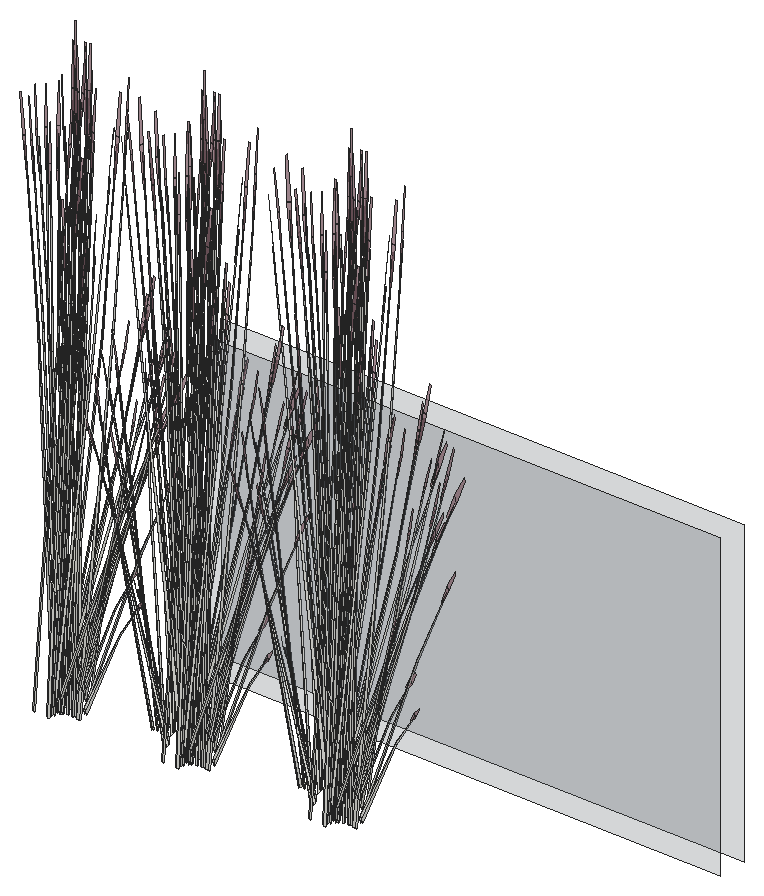
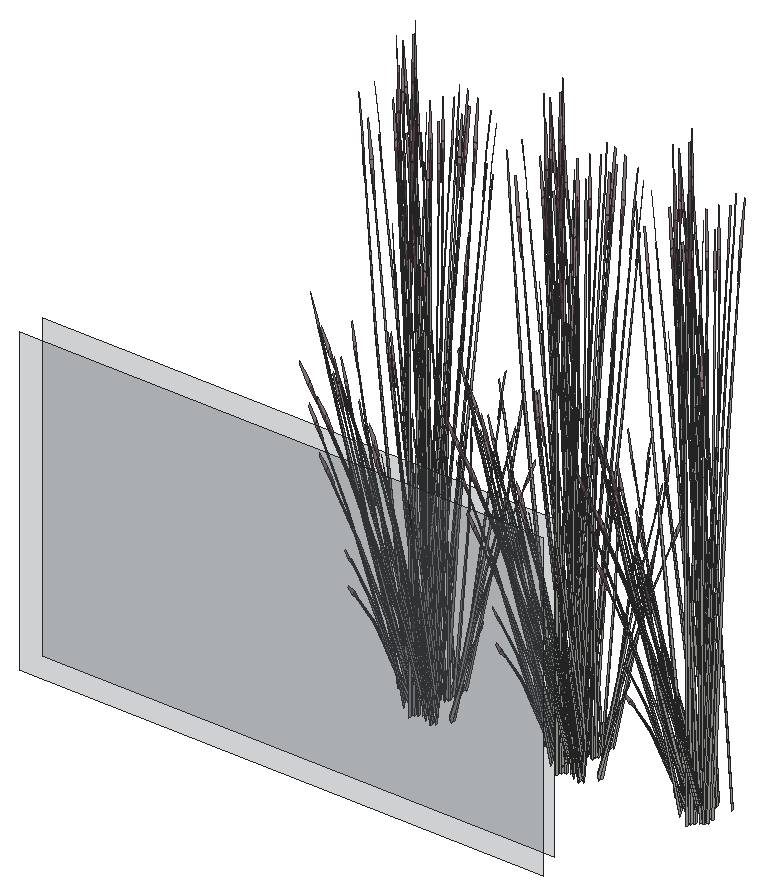
# SketchUp Ruby script. Lengths in inches.
U = 1.inch
M = Sketchup.active_model
def pt(a) = Geom::Point3d.new(a.map { |v| v * U })
def face(e, loops, mat)
  f = e.add_face(loops[0].map { |a| pt(a) })
  loops[1..].each { |l| e.add_face(l.map { |a| pt(a) }).erase! }
  f.material = f.back_material = mat if mat
  f
end
# faces: each face lists its corners as indices into pts; further lists are holes
def faces(e, pts, list, mat = nil) = list.each { |f| face(e, (f[0].is_a?(Array) ? f : [f]).map { |l| l.map { |i| pts[i] } }, mat) }
# xy, xz, yz: faces in a plane at the given z, y or x. An outline is a flat list of corners, or four numbers for a rectangle; further outlines are holes
def ring(l) = l.size == 4 ? [[l[0], l[1]], [l[2], l[1]], [l[2], l[3]], [l[0], l[3]]] : l.each_slice(2).to_a
def flat(e, list, mat, &to3) = list.each { |f| face(e, (f[0].is_a?(Array) ? f : [f]).map { |l| ring(l).map { |u, v| to3.(u, v) } }, mat) }
def xy(e, z, list, mat = nil) = flat(e, list, mat) { |x, y| [x, y, z] }
def xz(e, y, list, mat = nil) = flat(e, list, mat) { |x, z| [x, y, z] }
def yz(e, x, list, mat = nil) = flat(e, list, mat) { |y, z| [x, y, z] }
def lines(e, pts, list) = list.each { |a, b| e.add_line(pt(pts[a]), pt(pts[b])) }
# prism: a flat outline (further loops are holes) pulled along v
def prism(e, loops, v, mat = nil)
  f = face(e, loops, mat); d = Geom::Vector3d.new(v.map { |x| x * U })
  f.pushpull(f.normal.samedirection?(d) ? d.length : -d.length)
end
def box(e, o, s, mat = nil) = prism(e, [[o, [o[0] + s[0], o[1], o[2]], [o[0] + s[0], o[1] + s[1], o[2]], [o[0], o[1] + s[1], o[2]]]], [0, 0, s[2]], mat)
def at(x, y, z, deg = 0) = Geom::Transformation.translation(pt([x, y, z])) * Geom::Transformation.rotation(ORIGIN, Z_AXIS, deg.degrees)
def axes(o, x, y, z) = Geom::Transformation.new([*x, 0, *y, 0, *z, 0, *pt(o).to_a, 1])
def part(name) = M.definitions.add(name)
# library, detail: a bought-in or finely detailed component or shape, given as its bounding box
def library(name, o, s) = part(name).tap { |d| box(d.entities, o, s) }
def detail(e, o, s) = box(e.add_group.entities, o, s)
def put(e, d, t, mat = nil) = e.add_instance(d, t).tap { |i| i.material = mat if mat }
def group(e, t, mat = nil) = e.add_group.tap { |g| g.transformation = t; g.material = mat if mat }.entities
root = M.entities
M.materials.add("Glass_Basic_01").color = [105, 113, 122]
M.materials["Glass_Basic_01"].alpha = 0.25
M.materials.add("LightPink_Translucent").color = [144, 107, 117]
M.materials["LightPink_Translucent"].alpha = 0.75
c1 = part("blade")
p = [[2.15,0.21,22],[0,0.17,0],[0.09,0.45,0],[2.18,0.31,22],[2.29,0.31,22],[0.38,0.45,0],
  [2.48,0.24,33],[2.49,0.24,33],[2.48,0.22,33]]
faces(c1.entities,p,[[0,1,2,3],[4,5,2,3],[6,3,4,7],[8,0,3,6]])
c2 = part("seeds")
p = [[0.3,-0.1,1.38],[-0.01,-0.03,1.59],[-0.01,-0.03,0.03],[0.14,-0.07,-0.07],[0.29,-0.03,3],[0.15,0.01,3.11]]
faces(c2.entities,p,[[0,1,2,3],[1,0,4,5]],"LightPink_Translucent")
c3 = part("blade with seeds")
put(c3.entities,c1,at(0,0,0))
put(c3.entities,c2,axes([2.4,0.25,30.99],[1.5799,-0.05474,1.17369],[-0.12525,1.92788,0.29478],[-0.07173,-0.02425,1.56792]))
xz(root,474,[[275.49,398,329.45,430]],"Glass_Basic_01")
xz(root,477,[[274.25,398,329.5,430]],"Glass_Basic_01")
put(root,c3,axes([268.9,461.26,398.36],[0.63506,0.11347,0.45755],[-0.12924,0.64083,0.17955],[-0.09281,-0.06188,1.58856]))
put(root,c3,axes([268.56,462.28,398.47],[0.53992,-0.14294,0.17642],[0.13332,0.53195,0.35086],[-0.04815,-0.07751,1.60407]))
put(root,c3,axes([269.25,462.37,398.2],[-0.50654,-0.24178,0],[0.24378,-0.50239,0],[0,0,1.62707]))
put(root,c3,axes([270.43,462.97,398.375],[0.31414,0.53965,0],[-0.52557,0.30095,-0.51607],[-0.1197,0.06854,1.63711]))
put(root,c3,axes([270.17,462.3125,398.47],[0.14515,-0.53522,0.17642],[0.53115,0.15146,0.35086],[-0.09175,0.00261,1.60407]))
put(root,c3,axes([269.92,461.6,398.62],[0.37121,0.32357,0.1448],[-0.30963,0.36505,-0.41347],[-0.08619,0.04935,1.26744]))
put(root,c3,axes([269.91,461.37,398.72],[0.54562,-0.03324,0.44739],[0.04934,0.55185,-0.21531],[-0.09768,0.05593,1.43643]))
put(root,c3,axes([270.04,462.63,398.33],[0.62903,0.17504,0.30756],[-0.15737,0.62568,-0.36492],[-0.10411,0.07831,1.64885]))
put(root,c3,axes([270.32,462.6,398.48],[0.47024,-0.26927,0.49651],[0.28107,0.48284,0],[-0.1071,0.06133,1.57504]))
put(root,c3,axes([269.37,462.16,398.2],[-0.16394,-0.4643,0],[0.46814,-0.1626,0],[0,0,1.54371]))
put(root,c3,axes([268.88,463.3,400.53],[-0.15148,0.41415,-0.35414],[-0.44193,-0.12079,0.4572],[0.04052,0.16674,0.87481]))
put(root,c3,axes([271,460.95,398.47],[-0.39477,-0.39228,0.17642],[0.39783,-0.38049,0.35086],[-0.0436,0.08011,1.60407]))
put(root,c3,axes([269.95,460.97,398.29],[0,0.62282,-0.05637],[-0.62828,0,0],[0,0.01957,1.79368]))
put(root,c3,axes([268.61,459.52,398.47],[-0.14515,0.53522,0.17642],[-0.53115,-0.15146,0.35086],[0.09175,-0.00261,1.60407]))
put(root,c3,axes([269.65,462.18,398.29],[0.21845,0.61869,-0.06012],[-0.62418,0.21679,0],[0.00763,0.02161,1.72173]))
put(root,c3,axes([268.93,462.93,400.98],[0.23981,0.43789,-0.71045],[-0.49365,0.24404,0.08574],[0.05608,0.21158,1.00501]))
put(root,c3,axes([271.45,461.36,398.2],[-0.62797,-0.00431,-0.04976],[0,-0.6019,0.49943],[-0.01973,0.13702,1.58352]))
put(root,c3,axes([270.22,459.55,398.47],[-0.53992,0.14294,0.17642],[-0.13332,-0.53195,0.35086],[0.04815,0.07751,1.60407]))
put(root,c3,axes([270.05,461.1,398.21],[0.35073,0.34786,0],[-0.35073,0.34786,0],[0,0,1.69266]))
put(root,c3,axes([270.04,460.69,398.72],[0.24378,-0.48527,0.44739],[0.50654,0.23354,-0.21531],[0,0.11186,1.43643]))
put(root,c3,axes([269.83,462.38,398.2],[0.50654,0.24178,0],[-0.24378,0.50239,0],[0,0,1.74954]))
put(root,c3,axes([269.11,463.02,400.68],[0.49392,0.135,-0.51099],[-0.1693,0.46287,-0.3958],[0.04529,0.18636,0.97773]))
put(root,c3,axes([269.875,460.58,398.38],[-0.63506,-0.11347,0.49198],[0.12924,-0.64083,0.19306],[0.09281,0.06188,1.70813]))
put(root,c3,axes([270.06,460.86,398.21],[0.56215,0,0],[0,0.55754,0],[0,0,1.78407]))
put(root,c3,axes([269.52,460.25,398.72],[-0.30184,-0.45202,0.44739],[0.45719,-0.31831,-0.21531],[0.09768,0.05593,1.43643]))
put(root,c3,axes([270.25,460.8,398.62],[0.46814,-0.15705,0.1448],[0.16394,0.44848,-0.41347],[0,0.0987,1.26744]))
put(root,c3,axes([270.09,460.84,398.67],[0.56585,0.25696,-0.29095],[-0.27246,0.54236,-0.50002],[0.01778,0.13316,1.59708]))
put(root,c3,axes([271.32,460.96,398.48],[0,-0.53854,0.49651],[0.56215,0,0],[0,0.12266,1.57504]))
put(root,c3,axes([269.39,462.0625,399.875],[-0.11485,-0.17291,1.71376],[0.53072,-0.14557,0.13857],[0.11995,0.27145,0.73262]))
put(root,c3,axes([269.72,460.12,398.62],[0.09693,-0.48062,0.1448],[0.47357,0.08343,-0.41347],[0.08619,0.04935,1.26744]))
put(root,c3,axes([269.98,462.09,398.18],[0.5275,-0.18273,-0.19198],[0.18536,0.52636,0.00008],[0.05823,-0.0202,1.73897]))
put(root,c3,axes([270.85,462.58,398.77],[-0.2829,-0.15485,1.1486],[0.36529,-0.15734,0.84392],[0.09853,0.13328,0.25299]))
put(root,c3,axes([269.84,462.41,398.59],[0.00887,-0.17852,1.43002],[0.42372,-0.19941,-0.30754],[0.1308,0.21367,0.61141]))
put(root,c3,axes([271.7,461.05,398.375],[0.62828,0,0],[0,0.6019,-0.51607],[0,0.13709,1.63711]))
put(root,c3,axes([269.67,460.27,398.67],[0.5073,-0.35754,-0.29095],[0.33735,0.5052,-0.50002],[0.12516,0.05131,1.59708]))
put(root,c3,axes([270.89,463.28,398.67],[-0.3222,-0.01689,1.0506],[0.21278,-0.35872,0.58006],[0.12729,0.12745,0.8241]))
put(root,c3,axes([270.21,462.79,400.68],[0.4958,-0.12802,-0.51099],[0.08673,0.48481,-0.3958],[0.13317,0.13893,0.97773]))
put(root,c3,axes([272.03,462.4375,399.93],[-0.09617,-0.45271,-0.03492],[0.45453,-0.10408,-0.15832],[0.09492,0.0287,0.52218]))
put(root,c3,axes([270.16,461.52,399.875],[-0.18664,-0.09279,1.71376],[0.38624,-0.38925,0.13857],[0.24072,0.1756,0.73262]))
put(root,c3,axes([271.18,462.39,400.53],[0.28589,0.33718,-0.35414],[-0.32644,0.31919,0.4572],[0.16586,0.04856,0.87481]))
put(root,c3,axes([272.57,461.31,398.77],[-0.31044,0.08891,1.1486],[0.14613,-0.36744,0.84392],[0.16469,0.02514,0.25299]))
put(root,c3,axes([271.6875,461.22,400.53],[0.41757,0.15024,-0.35414],[-0.12179,0.4383,0.4572],[0.16812,-0.04019,0.87481]))
put(root,c3,axes([270.88,462.16,400.98],[0.50227,0.01297,-0.71045],[-0.03373,0.54602,0.08574],[0.21278,0.05762,1.00501]))
put(root,c3,axes([270.55,460.67,399.875],[-0.20841,0.0122,1.71376],[0.13825,-0.52864,0.13857],[0.297,0.0327,0.73262]))
put(root,c3,axes([280.66,461,399.875],[0.17434,-0.11391,1.71376],[0.14677,0.52637,0.13857],[-0.27369,0.11897,0.73262]))
put(root,c3,axes([280.12,461.89,398.59],[0.17462,0.04421,1.43002],[0.11254,0.45156,-0.30754],[-0.23719,0.08453,0.61141]))
put(root,c3,axes([281.67,460.45,399.34],[0.14282,-0.0779,1.77064],[0.04925,0.54394,0.13857],[-0.30935,0.07218,0.63284]))
put(root,c3,axes([271.99,461.9,398.59],[-0.12101,-0.13245,1.43002],[0.15744,-0.43816,-0.30754],[0.24483,0.05936,0.61141]))
put(root,c3,axes([280.39,460.52,400.53],[-0.41757,-0.15024,-0.35414],[0.12179,-0.4383,0.4572],[-0.16812,0.04019,0.87481]))
put(root,c3,axes([280.68,460.74,400.68],[-0.13612,0.48987,-0.51099],[-0.46669,-0.16791,-0.3958],[-0.1879,0.04492,0.97773]))
put(root,c3,axes([279.76,462.84,398.77],[0.2094,-0.24408,1.1486],[0.08263,0.38639,0.84392],[-0.15132,0.06919,0.25299]))
put(root,c3,axes([281.3,461.35,399.875],[0.1255,-0.16547,1.71376],[0.31687,0.44665,0.13857],[-0.21734,0.2034,0.73262]))
put(root,c3,axes([280.55,461.78,400.53],[-0.43736,0.07697,-0.35414],[-0.11549,-0.43998,0.4572],[-0.12533,0.11818,0.87481]))
put(root,c3,axes([281.21,461.76,399.875],[0.09355,-0.18511,1.71376],[0.39247,0.38307,0.13857],[-0.17705,0.23875,0.73262]))
put(root,c3,axes([280.91,461.83,400.68],[0.12908,0.49174,-0.51099],[-0.48882,0.08602,-0.3958],[-0.14008,0.13208,0.97773]))
put(root,c3,axes([281.73,462.84,398.375],[-0.31414,0.53965,0],[-0.52557,-0.30095,-0.51607],[-0.1197,-0.06854,1.63711]))
put(root,c3,axes([281.15,463.62,398.59],[0.15856,-0.08496,1.43002],[0.39147,0.25616,-0.30754],[-0.11652,0.22165,0.61141]))
put(root,c3,axes([282.72,461.5625,398.67],[-0.5073,0.35754,-0.29095],[-0.33735,-0.5052,-0.50002],[-0.12516,-0.05131,1.59708]))
put(root,c3,axes([281.32,462.8,400.53],[-0.33997,0.28354,-0.35414],[-0.32182,-0.32376,0.4572],[-0.04897,0.1645,0.87481]))
put(root,c3,axes([283.29,461.73,398.46],[-0.49063,-0.43346,-0.25192],[0.41285,-0.48673,0.5513],[-0.13212,0.05071,1.68216]))
put(root,c3,axes([281.54,462.5,401.34],[-0.01307,0.49815,-0.7886],[-0.55054,-0.03346,0.09517],[-0.0581,0.21104,1.11556]))
put(root,c3,axes([281.53,463.9,398.77],[-0.013,-0.32022,1.1486],[0.32493,0.22839,0.84392],[-0.0639,0.15263,0.25299]))
put(root,c3,axes([282,462.56,398.48],[0.47024,0.26927,0.49651],[-0.28107,0.48284,0],[-0.1071,-0.06133,1.57504]))
put(root,c3,axes([281.36,463.2,399.36],[0.01104,-0.27801,1.54345],[0.49652,0.14685,0.21329],[-0.04302,0.2963,0.72882]))
put(root,c3,axes([282.67,461.72,398.62],[-0.09693,0.48062,0.1448],[-0.47357,-0.08343,-0.41347],[-0.08619,-0.04935,1.26744]))
put(root,c3,axes([283.64,462.91,398.19],[-0.31023,-0.54153,-0.05142],[0.52557,-0.30095,0.51607],[-0.12951,0.05156,1.6363]))
put(root,c3,axes([281.65,462.67,401],[0.35968,0.36185,-0.5672],[-0.37996,0.3169,-0.43934],[-0.05473,0.18385,1.08528]))
put(root,c3,axes([283.77,460.84,398.84],[-0.01373,-0.50706,1.41272],[0.62119,0.13144,0.59816],[-0.14692,0.27746,1.3335]))
put(root,c3,axes([281.26,463.21,398.82],[0.45645,-0.09537,0.06507],[0.10494,0.38421,-0.86304],[-0.02894,0.19449,0.7736]))
put(root,c3,axes([283.42,461.48,398.67],[0.05855,0.61451,-0.29095],[-0.60981,0.03716,-0.50002],[-0.10738,0.08185,1.59708]))
put(root,c3,axes([282.0625,462.15,399.875],[-0.0123,-0.2067,1.71376],[0.53301,0.13712,0.13857],[-0.03297,0.29456,0.73262]))
put(root,c3,axes([282.51,461.26,398.36],[0.63506,0.11347,0.45755],[-0.12924,0.64083,0.17955],[-0.09281,-0.06188,1.58856]))
put(root,c3,axes([282.17,462.28,398.47],[0.53992,-0.14294,0.17642],[0.13332,0.53195,0.35086],[-0.04815,-0.07751,1.60407]))
put(root,c3,axes([282.87,462.37,398.2],[-0.50654,-0.24178,0],[0.24378,-0.50239,0],[0,0,1.62707]))
put(root,c3,axes([284.04,462.97,398.375],[0.31414,0.53965,0],[-0.52557,0.30095,-0.51607],[-0.1197,0.06854,1.63711]))
put(root,c3,axes([283.78,462.3125,398.47],[0.14515,-0.53522,0.17642],[0.53115,0.15146,0.35086],[-0.09175,0.00261,1.60407]))
put(root,c3,axes([283.53,461.6,398.62],[0.37121,0.32357,0.1448],[-0.30963,0.36505,-0.41347],[-0.08619,0.04935,1.26744]))
put(root,c3,axes([283.53,461.37,398.72],[0.54562,-0.03324,0.44739],[0.04934,0.55185,-0.21531],[-0.09768,0.05593,1.43643]))
put(root,c3,axes([283.66,462.63,398.33],[0.62903,0.17504,0.30756],[-0.15737,0.62568,-0.36492],[-0.10411,0.07831,1.64885]))
put(root,c3,axes([283.93,462.6,398.48],[0.47024,-0.26927,0.49651],[0.28107,0.48284,0],[-0.1071,0.06133,1.57504]))
put(root,c3,axes([282.98,462.16,398.2],[-0.16394,-0.4643,0],[0.46814,-0.1626,0],[0,0,1.54371]))
put(root,c3,axes([282.5,463.3,400.53],[-0.15148,0.41415,-0.35414],[-0.44193,-0.12079,0.4572],[0.04052,0.16674,0.87481]))
put(root,c3,axes([284.61,460.95,398.47],[-0.39477,-0.39228,0.17642],[0.39783,-0.38049,0.35086],[-0.0436,0.08011,1.60407]))
put(root,c3,axes([283.5625,460.97,398.29],[0,0.62282,-0.05637],[-0.62828,0,0],[0,0.01957,1.79368]))
put(root,c3,axes([282.22,459.52,398.47],[-0.14515,0.53522,0.17642],[-0.53115,-0.15146,0.35086],[0.09175,-0.00261,1.60407]))
put(root,c3,axes([283.26,462.18,398.29],[0.21845,0.61869,-0.06012],[-0.62418,0.21679,0],[0.00763,0.02161,1.72173]))
put(root,c3,axes([282.54,462.93,400.98],[0.23981,0.43789,-0.71045],[-0.49365,0.24404,0.08574],[0.05608,0.21158,1.00501]))
put(root,c3,axes([285.0625,461.36,398.2],[-0.62797,-0.00431,-0.04976],[0,-0.6019,0.49943],[-0.01973,0.13702,1.58352]))
put(root,c3,axes([283.83,459.55,398.47],[-0.53992,0.14294,0.17642],[-0.13332,-0.53195,0.35086],[0.04815,0.07751,1.60407]))
put(root,c3,axes([283.66,461.1,398.21],[0.35073,0.34786,0],[-0.35073,0.34786,0],[0,0,1.69266]))
put(root,c3,axes([283.65,460.69,398.72],[0.24378,-0.48527,0.44739],[0.50654,0.23354,-0.21531],[0,0.11186,1.43643]))
put(root,c3,axes([283.44,462.38,398.2],[0.50654,0.24178,0],[-0.24378,0.50239,0],[0,0,1.74954]))
put(root,c3,axes([282.72,463.02,400.68],[0.49392,0.135,-0.51099],[-0.1693,0.46287,-0.3958],[0.04529,0.18636,0.97773]))
put(root,c3,axes([283.49,460.58,398.38],[-0.63506,-0.11347,0.49198],[0.12924,-0.64083,0.19306],[0.09281,0.06188,1.70813]))
put(root,c3,axes([283.67,460.86,398.21],[0.56215,0,0],[0,0.55754,0],[0,0,1.78407]))
put(root,c3,axes([283.13,460.25,398.72],[-0.30184,-0.45202,0.44739],[0.45719,-0.31831,-0.21531],[0.09768,0.05593,1.43643]))
put(root,c3,axes([283.87,460.8,398.62],[0.46814,-0.15705,0.1448],[0.16394,0.44848,-0.41347],[0,0.0987,1.26744]))
put(root,c3,axes([283.71,460.84,398.67],[0.56585,0.25696,-0.29095],[-0.27246,0.54236,-0.50002],[0.01778,0.13316,1.59708]))
put(root,c3,axes([284.93,460.96,398.48],[0,-0.53854,0.49651],[0.56215,0,0],[0,0.12266,1.57504]))
put(root,c3,axes([283,462.0625,399.875],[-0.11485,-0.17291,1.71376],[0.53072,-0.14557,0.13857],[0.11995,0.27145,0.73262]))
put(root,c3,axes([283.33,460.12,398.62],[0.09693,-0.48062,0.1448],[0.47357,0.08343,-0.41347],[0.08619,0.04935,1.26744]))
put(root,c3,axes([283.6,462.09,398.18],[0.5275,-0.18273,-0.19198],[0.18536,0.52636,0.00008],[0.05823,-0.0202,1.73897]))
put(root,c3,axes([284.46,462.58,398.77],[-0.2829,-0.15485,1.1486],[0.36529,-0.15734,0.84392],[0.09853,0.13328,0.25299]))
put(root,c3,axes([283.45,462.41,398.59],[0.00887,-0.17852,1.43002],[0.42372,-0.19941,-0.30754],[0.1308,0.21367,0.61141]))
put(root,c3,axes([285.32,461.05,398.375],[0.62828,0,0],[0,0.6019,-0.51607],[0,0.13709,1.63711]))
put(root,c3,axes([283.28,460.27,398.67],[0.5073,-0.35754,-0.29095],[0.33735,0.5052,-0.50002],[0.12516,0.05131,1.59708]))
put(root,c3,axes([284.51,463.28,398.67],[-0.3222,-0.01689,1.0506],[0.21278,-0.35872,0.58006],[0.12729,0.12745,0.8241]))
put(root,c3,axes([283.82,462.79,400.68],[0.4958,-0.12802,-0.51099],[0.08673,0.48481,-0.3958],[0.13317,0.13893,0.97773]))
put(root,c3,axes([285.65,462.4375,399.93],[-0.09617,-0.45271,-0.03492],[0.45453,-0.10408,-0.15832],[0.09492,0.0287,0.52218]))
put(root,c3,axes([283.77,461.52,399.875],[-0.18664,-0.09279,1.71376],[0.38624,-0.38925,0.13857],[0.24072,0.1756,0.73262]))
put(root,c3,axes([284.8,462.39,400.53],[0.28589,0.33718,-0.35414],[-0.32644,0.31919,0.4572],[0.16586,0.04856,0.87481]))
put(root,c3,axes([286.1875,461.31,398.77],[-0.31044,0.08891,1.1486],[0.14613,-0.36744,0.84392],[0.16469,0.02514,0.25299]))
put(root,c3,axes([285.3,461.22,400.53],[0.41757,0.15024,-0.35414],[-0.12179,0.4383,0.4572],[0.16812,-0.04019,0.87481]))
put(root,c3,axes([284.49,462.16,400.98],[0.50227,0.01297,-0.71045],[-0.03373,0.54602,0.08574],[0.21278,0.05762,1.00501]))
put(root,c3,axes([284.16,460.67,399.875],[-0.20841,0.0122,1.71376],[0.13825,-0.52864,0.13857],[0.297,0.0327,0.73262]))
put(root,c3,axes([285.61,461.9,398.59],[-0.12101,-0.13245,1.43002],[0.15744,-0.43816,-0.30754],[0.24483,0.05936,0.61141]))
put(root,c3,axes([296.19,461,399.875],[0.17434,-0.11391,1.71376],[0.14677,0.52637,0.13857],[-0.27369,0.11897,0.73262]))
put(root,c3,axes([295.65,461.89,398.59],[0.17462,0.04421,1.43002],[0.11254,0.45156,-0.30754],[-0.23719,0.08453,0.61141]))
put(root,c3,axes([297.2,460.45,399.34],[0.14282,-0.0779,1.77064],[0.04925,0.54394,0.13857],[-0.30935,0.07218,0.63284]))
put(root,c3,axes([295.92,460.52,400.53],[-0.41757,-0.15024,-0.35414],[0.12179,-0.4383,0.4572],[-0.16812,0.04019,0.87481]))
put(root,c3,axes([296.21,460.74,400.68],[-0.13612,0.48987,-0.51099],[-0.46669,-0.16791,-0.3958],[-0.1879,0.04492,0.97773]))
put(root,c3,axes([295.29,462.84,398.77],[0.2094,-0.24408,1.1486],[0.08263,0.38639,0.84392],[-0.15132,0.06919,0.25299]))
put(root,c3,axes([296.83,461.35,399.875],[0.1255,-0.16547,1.71376],[0.31687,0.44665,0.13857],[-0.21734,0.2034,0.73262]))
put(root,c3,axes([296.08,461.78,400.53],[-0.43736,0.07697,-0.35414],[-0.11549,-0.43998,0.4572],[-0.12533,0.11818,0.87481]))
put(root,c3,axes([296.74,461.76,399.875],[0.09355,-0.18511,1.71376],[0.39247,0.38307,0.13857],[-0.17705,0.23875,0.73262]))
put(root,c3,axes([296.4375,461.83,400.68],[0.12908,0.49174,-0.51099],[-0.48882,0.08602,-0.3958],[-0.14008,0.13208,0.97773]))
put(root,c3,axes([297.26,462.84,398.375],[-0.31414,0.53965,0],[-0.52557,-0.30095,-0.51607],[-0.1197,-0.06854,1.63711]))
put(root,c3,axes([296.68,463.62,398.59],[0.15856,-0.08496,1.43002],[0.39147,0.25616,-0.30754],[-0.11652,0.22165,0.61141]))
put(root,c3,axes([298.25,461.5625,398.67],[-0.5073,0.35754,-0.29095],[-0.33735,-0.5052,-0.50002],[-0.12516,-0.05131,1.59708]))
put(root,c3,axes([296.85,462.8,400.53],[-0.33997,0.28354,-0.35414],[-0.32182,-0.32376,0.4572],[-0.04897,0.1645,0.87481]))
put(root,c3,axes([298.82,461.73,398.46],[-0.49063,-0.43346,-0.25192],[0.41285,-0.48673,0.5513],[-0.13212,0.05071,1.68216]))
put(root,c3,axes([297.07,462.5,401.34],[-0.01307,0.49815,-0.7886],[-0.55054,-0.03346,0.09517],[-0.0581,0.21104,1.11556]))
put(root,c3,axes([297.0625,463.9,398.77],[-0.013,-0.32022,1.1486],[0.32493,0.22839,0.84392],[-0.0639,0.15263,0.25299]))
put(root,c3,axes([297.53,462.56,398.48],[0.47024,0.26927,0.49651],[-0.28107,0.48284,0],[-0.1071,-0.06133,1.57504]))
put(root,c3,axes([296.89,463.2,399.36],[0.01104,-0.27801,1.54345],[0.49652,0.14685,0.21329],[-0.04302,0.2963,0.72882]))
put(root,c3,axes([298.2,461.72,398.62],[-0.09693,0.48062,0.1448],[-0.47357,-0.08343,-0.41347],[-0.08619,-0.04935,1.26744]))
put(root,c3,axes([299.17,462.91,398.19],[-0.31023,-0.54153,-0.05142],[0.52557,-0.30095,0.51607],[-0.12951,0.05156,1.6363]))
put(root,c3,axes([297.18,462.67,401],[0.35968,0.36185,-0.5672],[-0.37996,0.3169,-0.43934],[-0.05473,0.18385,1.08528]))
put(root,c3,axes([299.3,460.84,398.84],[-0.01373,-0.50706,1.41272],[0.62119,0.13144,0.59816],[-0.14692,0.27746,1.3335]))
put(root,c3,axes([296.79,463.21,398.82],[0.45645,-0.09537,0.06507],[0.10494,0.38421,-0.86304],[-0.02894,0.19449,0.7736]))
put(root,c3,axes([298.95,461.48,398.67],[0.05855,0.61451,-0.29095],[-0.60981,0.03716,-0.50002],[-0.10738,0.08185,1.59708]))
put(root,c3,axes([297.59,462.15,399.875],[-0.0123,-0.2067,1.71376],[0.53301,0.13712,0.13857],[-0.03297,0.29456,0.73262]))
put(root,c3,axes([298.04,461.26,398.36],[0.63506,0.11347,0.45755],[-0.12924,0.64083,0.17955],[-0.09281,-0.06188,1.58856]))
put(root,c3,axes([297.7,462.28,398.47],[0.53992,-0.14294,0.17642],[0.13332,0.53195,0.35086],[-0.04815,-0.07751,1.60407]))
put(root,c3,axes([298.4,462.37,398.2],[-0.50654,-0.24178,0],[0.24378,-0.50239,0],[0,0,1.62707]))
put(root,c3,axes([299.57,462.97,398.375],[0.31414,0.53965,0],[-0.52557,0.30095,-0.51607],[-0.1197,0.06854,1.63711]))
put(root,c3,axes([299.31,462.3125,398.47],[0.14515,-0.53522,0.17642],[0.53115,0.15146,0.35086],[-0.09175,0.00261,1.60407]))
put(root,c3,axes([299.0625,461.6,398.62],[0.37121,0.32357,0.1448],[-0.30963,0.36505,-0.41347],[-0.08619,0.04935,1.26744]))
put(root,c3,axes([299.06,461.37,398.72],[0.54562,-0.03324,0.44739],[0.04934,0.55185,-0.21531],[-0.09768,0.05593,1.43643]))
put(root,c3,axes([299.1875,462.63,398.33],[0.62903,0.17504,0.30756],[-0.15737,0.62568,-0.36492],[-0.10411,0.07831,1.64885]))
put(root,c3,axes([299.46,462.6,398.48],[0.47024,-0.26927,0.49651],[0.28107,0.48284,0],[-0.1071,0.06133,1.57504]))
put(root,c3,axes([298.51,462.16,398.2],[-0.16394,-0.4643,0],[0.46814,-0.1626,0],[0,0,1.54371]))
put(root,c3,axes([298.03,463.3,400.53],[-0.15148,0.41415,-0.35414],[-0.44193,-0.12079,0.4572],[0.04052,0.16674,0.87481]))
put(root,c3,axes([300.14,460.95,398.47],[-0.39477,-0.39228,0.17642],[0.39783,-0.38049,0.35086],[-0.0436,0.08011,1.60407]))
put(root,c3,axes([299.09,460.97,398.29],[0,0.62282,-0.05637],[-0.62828,0,0],[0,0.01957,1.79368]))
put(root,c3,axes([297.75,459.52,398.47],[-0.14515,0.53522,0.17642],[-0.53115,-0.15146,0.35086],[0.09175,-0.00261,1.60407]))
put(root,c3,axes([298.79,462.18,398.29],[0.21845,0.61869,-0.06012],[-0.62418,0.21679,0],[0.00763,0.02161,1.72173]))
put(root,c3,axes([298.07,462.93,400.98],[0.23981,0.43789,-0.71045],[-0.49365,0.24404,0.08574],[0.05608,0.21158,1.00501]))
put(root,c3,axes([300.59,461.36,398.2],[-0.62797,-0.00431,-0.04976],[0,-0.6019,0.49943],[-0.01973,0.13702,1.58352]))
put(root,c3,axes([299.36,459.55,398.47],[-0.53992,0.14294,0.17642],[-0.13332,-0.53195,0.35086],[0.04815,0.07751,1.60407]))
put(root,c3,axes([299.1875,461.1,398.21],[0.35073,0.34786,0],[-0.35073,0.34786,0],[0,0,1.69266]))
put(root,c3,axes([299.18,460.69,398.72],[0.24378,-0.48527,0.44739],[0.50654,0.23354,-0.21531],[0,0.11186,1.43643]))
put(root,c3,axes([298.97,462.38,398.2],[0.50654,0.24178,0],[-0.24378,0.50239,0],[0,0,1.74954]))
put(root,c3,axes([298.25,463.02,400.68],[0.49392,0.135,-0.51099],[-0.1693,0.46287,-0.3958],[0.04529,0.18636,0.97773]))
put(root,c3,axes([299.02,460.58,398.38],[-0.63506,-0.11347,0.49198],[0.12924,-0.64083,0.19306],[0.09281,0.06188,1.70813]))
put(root,c3,axes([299.2,460.86,398.21],[0.56215,0,0],[0,0.55754,0],[0,0,1.78407]))
put(root,c3,axes([298.66,460.25,398.72],[-0.30184,-0.45202,0.44739],[0.45719,-0.31831,-0.21531],[0.09768,0.05593,1.43643]))
put(root,c3,axes([299.4,460.8,398.62],[0.46814,-0.15705,0.1448],[0.16394,0.44848,-0.41347],[0,0.0987,1.26744]))
put(root,c3,axes([299.24,460.84,398.67],[0.56585,0.25696,-0.29095],[-0.27246,0.54236,-0.50002],[0.01778,0.13316,1.59708]))
put(root,c3,axes([300.46,460.96,398.48],[0,-0.53854,0.49651],[0.56215,0,0],[0,0.12266,1.57504]))
put(root,c3,axes([298.53,462.0625,399.875],[-0.11485,-0.17291,1.71376],[0.53072,-0.14557,0.13857],[0.11995,0.27145,0.73262]))
put(root,c3,axes([298.86,460.12,398.62],[0.09693,-0.48062,0.1448],[0.47357,0.08343,-0.41347],[0.08619,0.04935,1.26744]))
put(root,c3,axes([299.125,462.09,398.18],[0.5275,-0.18273,-0.19198],[0.18536,0.52636,0.00008],[0.05823,-0.0202,1.73897]))
put(root,c3,axes([299.99,462.58,398.77],[-0.2829,-0.15485,1.1486],[0.36529,-0.15734,0.84392],[0.09853,0.13328,0.25299]))
put(root,c3,axes([298.98,462.41,398.59],[0.00887,-0.17852,1.43002],[0.42372,-0.19941,-0.30754],[0.1308,0.21367,0.61141]))
put(root,c3,axes([300.85,461.05,398.375],[0.62828,0,0],[0,0.6019,-0.51607],[0,0.13709,1.63711]))
put(root,c3,axes([298.81,460.27,398.67],[0.5073,-0.35754,-0.29095],[0.33735,0.5052,-0.50002],[0.12516,0.05131,1.59708]))
put(root,c3,axes([300.04,463.28,398.67],[-0.3222,-0.01689,1.0506],[0.21278,-0.35872,0.58006],[0.12729,0.12745,0.8241]))
put(root,c3,axes([299.35,462.79,400.68],[0.4958,-0.12802,-0.51099],[0.08673,0.48481,-0.3958],[0.13317,0.13893,0.97773]))
put(root,c3,axes([301.18,462.4375,399.93],[-0.09617,-0.45271,-0.03492],[0.45453,-0.10408,-0.15832],[0.09492,0.0287,0.52218]))
put(root,c3,axes([299.3,461.52,399.875],[-0.18664,-0.09279,1.71376],[0.38624,-0.38925,0.13857],[0.24072,0.1756,0.73262]))
put(root,c3,axes([300.33,462.39,400.53],[0.28589,0.33718,-0.35414],[-0.32644,0.31919,0.4572],[0.16586,0.04856,0.87481]))
put(root,c3,axes([301.72,461.31,398.77],[-0.31044,0.08891,1.1486],[0.14613,-0.36744,0.84392],[0.16469,0.02514,0.25299]))
put(root,c3,axes([300.83,461.22,400.53],[0.41757,0.15024,-0.35414],[-0.12179,0.4383,0.4572],[0.16812,-0.04019,0.87481]))
put(root,c3,axes([300.02,462.16,400.98],[0.50227,0.01297,-0.71045],[-0.03373,0.54602,0.08574],[0.21278,0.05762,1.00501]))
put(root,c3,axes([299.69,460.67,399.875],[-0.20841,0.0122,1.71376],[0.13825,-0.52864,0.13857],[0.297,0.0327,0.73262]))
put(root,c3,axes([301.14,461.9,398.59],[-0.12101,-0.13245,1.43002],[0.15744,-0.43816,-0.30754],[0.24483,0.05936,0.61141]))
